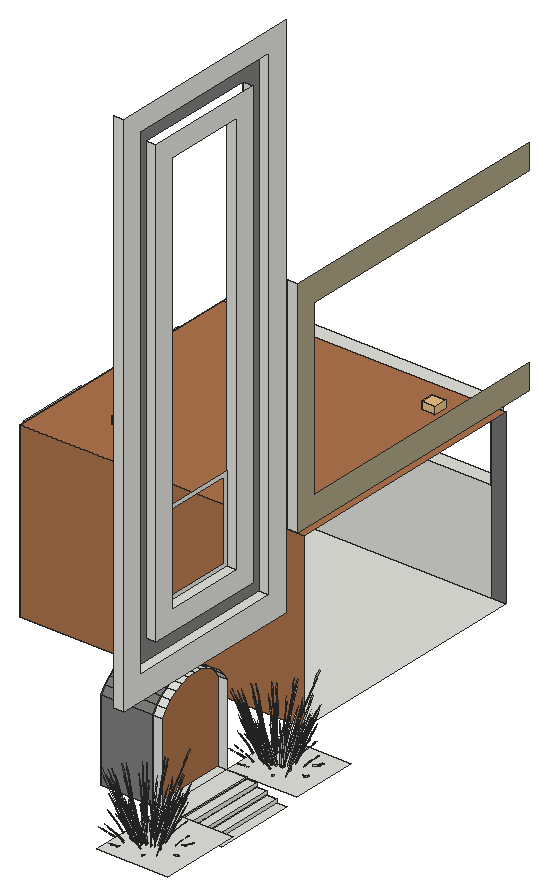
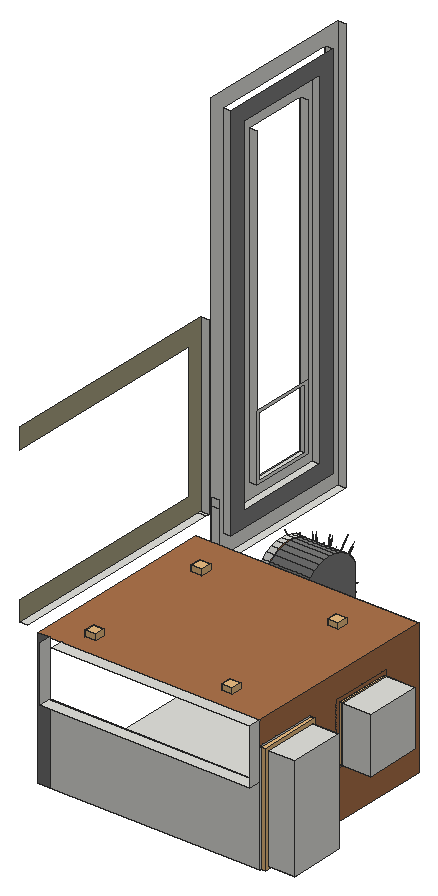
# SketchUp Ruby script. Lengths in inches.
U = 1.inch
M = Sketchup.active_model
def pt(a) = Geom::Point3d.new(a.map { |v| v * U })
def face(e, loops, mat)
  f = e.add_face(loops[0].map { |a| pt(a) })
  loops[1..].each { |l| e.add_face(l.map { |a| pt(a) }).erase! }
  f.material = f.back_material = mat if mat
  f
end
# faces: each face lists its corners as indices into pts; further lists are holes
def faces(e, pts, list, mat = nil) = list.each { |f| face(e, (f[0].is_a?(Array) ? f : [f]).map { |l| l.map { |i| pts[i] } }, mat) }
# xy, xz, yz: faces in a plane at the given z, y or x. An outline is a flat list of corners, or four numbers for a rectangle; further outlines are holes
def ring(l) = l.size == 4 ? [[l[0], l[1]], [l[2], l[1]], [l[2], l[3]], [l[0], l[3]]] : l.each_slice(2).to_a
def flat(e, list, mat, &to3) = list.each { |f| face(e, (f[0].is_a?(Array) ? f : [f]).map { |l| ring(l).map { |u, v| to3.(u, v) } }, mat) }
def xy(e, z, list, mat = nil) = flat(e, list, mat) { |x, y| [x, y, z] }
def xz(e, y, list, mat = nil) = flat(e, list, mat) { |x, z| [x, y, z] }
def yz(e, x, list, mat = nil) = flat(e, list, mat) { |y, z| [x, y, z] }
def lines(e, pts, list) = list.each { |a, b| e.add_line(pt(pts[a]), pt(pts[b])) }
# prism: a flat outline (further loops are holes) pulled along v
def prism(e, loops, v, mat = nil)
  f = face(e, loops, mat); d = Geom::Vector3d.new(v.map { |x| x * U })
  f.pushpull(f.normal.samedirection?(d) ? d.length : -d.length)
end
def box(e, o, s, mat = nil) = prism(e, [[o, [o[0] + s[0], o[1], o[2]], [o[0] + s[0], o[1] + s[1], o[2]], [o[0], o[1] + s[1], o[2]]]], [0, 0, s[2]], mat)
def at(x, y, z, deg = 0) = Geom::Transformation.translation(pt([x, y, z])) * Geom::Transformation.rotation(ORIGIN, Z_AXIS, deg.degrees)
def axes(o, x, y, z) = Geom::Transformation.new([*x, 0, *y, 0, *z, 0, *pt(o).to_a, 1])
def part(name) = M.definitions.add(name)
# library, detail: a bought-in or finely detailed component or shape, given as its bounding box
def library(name, o, s) = part(name).tap { |d| box(d.entities, o, s) }
def detail(e, o, s) = box(e.add_group.entities, o, s)
def put(e, d, t, mat = nil) = e.add_instance(d, t).tap { |i| i.material = mat if mat }
def group(e, t, mat = nil) = e.add_group.tap { |g| g.transformation = t; g.material = mat if mat }.entities
root = M.entities
M.materials.add("LightPink_Translucent").color = [144, 107, 117]
M.materials["LightPink_Translucent"].alpha = 0.75
M.materials.add("M05_Graphite_Haze").color = [114, 114, 114]
M.materials.add("ThomThom - Beard1").color = [170, 163, 131]
M.materials.add("ThomThom - Waistcoat2").color = [127, 127, 126]
M.materials.add("Wood_Veneer_15_1K").color = [173, 116, 75]
c1 = part("blade")
p = [[2.15,0.21,22],[0,0.17,0],[0.09,0.45,0],[2.18,0.31,22],[2.29,0.31,22],[0.38,0.45,0],
  [2.48,0.24,33],[2.49,0.24,33],[2.48,0.22,33]]
faces(c1.entities,p,[[0,1,2,3],[4,5,2,3],[6,3,4,7],[8,0,3,6]])
c2 = part("seeds")
p = [[0.3,-0.1,1.38],[-0.01,-0.03,1.59],[-0.01,-0.03,0.03],[0.14,-0.07,-0.07],[0.29,-0.03,3],[0.15,0.01,3.11]]
faces(c2.entities,p,[[0,1,2,3],[1,0,4,5]],"LightPink_Translucent")
c3 = part("blade with seeds")
put(c3.entities,c1,at(0,0,0))
put(c3.entities,c2,axes([2.4,0.25,30.99],[1.5799,-0.05474,1.17369],[-0.12525,1.92788,0.29478],[-0.07173,-0.02425,1.56792]))
c4 = library("porta+4",[0.2,-5.42,1.33],[46.55,4.72,83.21])
c5 = library("Group\#3",[0,0,0],[2.375,32.33,79.75])
c6 = library("Sphere Light\#7",[-4.125,-4.125,-4.125],[8.25,8.25,8.25])
c7 = library("Sphere Light\#8",[-4,-4,-4],[8,8,8])
c8 = library("Sphere Light\#9",[-4,-4,-4],[8,8,8])
c9 = library("Sphere Light\#10",[-4,-4,-4],[8,8,8])
xy(root,4.51,[[503.8,48,509.78,96],[509.78,48,515.75,96]])
xy(root,6.76,[[497.83,48,503.8,96],[503.8,48,509.78,96]])
xy(root,9,[[312,153,480,303]])
xy(root,9.01,[[491.86,48,497.83,96],[497.83,48,503.8,96]])
xy(root,11.26,[[480,48,491.86,96],[491.86,48,497.83,96]])
xy(root,12,[[480,0,521.72,0,521.72,48,491.86,48,491.86,96,480,96],[474.67,48,480,96],[480,96,521.72,136.05],[288,258,312,300]])
xy(root,12,[[444,48,474.67,96]],"ThomThom - Waistcoat2")
xy(root,48,[[288,186,312,228]])
xy(root,69,[[312,303,471,312]])
xy(root,81.33,[[480,12,486,132]])
xy(root,90,[[288,186,312,228],[288,258,312,300]])
xy(root,96,[[480,24,486,120]])
xy(root,108,[[480,36,486,108]])
xy(root,111,[[312,303,462,312]])
xy(root,111,[[[312,153,480,303],[348.15,280.73,349.1875,280.78,350.18,281.11,351.06,281.68,351.75,282.46,352.23,283.39,352.44,284.41,352.38,285.45,352.06,286.44,351.49,287.32,350.71,288.02,349.78,288.49,348.76,288.7,347.71,288.65,346.72,288.32,345.85,287.75,345.15,286.97,344.68,286.04,344.46,285.02,344.52,283.98,344.85,282.99,345.42,282.11,346.19,281.41,347.125,280.94],[348.15,180.38,349.1875,180.4375,350.18,180.76,351.06,181.33,351.75,182.11,352.23,183.04,352.44,184.06,352.38,185.11,352.06,186.1,351.49,186.97,350.71,187.67,349.78,188.14,348.76,188.36,347.71,188.3,346.72,187.98,345.85,187.41,345.15,186.63,344.68,185.7,344.46,184.68,344.52,183.63,344.85,182.64,345.42,181.77,346.19,181.07,347.125,180.6],[451.37,180.38,452.41,180.4375,453.4,180.76,454.28,181.33,454.97,182.11,455.45,183.04,455.66,184.06,455.61,185.11,455.28,186.1,454.71,186.97,453.93,187.67,453,188.14,451.98,188.36,450.9375,188.3,449.94,187.98,449.07,187.41,448.37,186.63,447.9,185.7,447.69,184.68,447.74,183.63,448.07,182.64,448.64,181.77,449.42,181.07,450.35,180.6],[451.37,280.73,452.41,280.78,453.4,281.11,454.28,281.68,454.97,282.46,455.45,283.39,455.66,284.41,455.61,285.45,455.28,286.44,454.71,287.32,453.93,288.02,453,288.49,451.98,288.7,450.9375,288.65,449.94,288.32,449.07,287.75,448.37,286.97,447.9,286.04,447.69,285.02,447.74,283.98,448.07,282.99,448.64,282.11,449.42,281.41,450.35,280.94]],[348.15,180.38,347.125,180.6,346.19,181.07,345.42,181.77,344.85,182.64,344.52,183.63,344.46,184.68,344.68,185.7,345.15,186.63,345.85,187.41,346.72,187.98,347.71,188.3,348.76,188.36,349.78,188.14,350.71,187.67,351.49,186.97,352.06,186.1,352.38,185.11,352.44,184.06,352.23,183.04,351.75,182.11,351.06,181.33,350.18,180.76,349.1875,180.4375],[451.37,180.38,450.35,180.6,449.42,181.07,448.64,181.77,448.07,182.64,447.74,183.63,447.69,184.68,447.9,185.7,448.37,186.63,449.07,187.41,449.94,187.98,450.9375,188.3,451.98,188.36,453,188.14,453.93,187.67,454.71,186.97,455.28,186.1,455.61,185.11,455.66,184.06,455.45,183.04,454.97,182.11,454.28,181.33,453.4,180.76,452.41,180.4375],[348.15,280.73,347.125,280.94,346.19,281.41,345.42,282.11,344.85,282.99,344.52,283.98,344.46,285.02,344.68,286.04,345.15,286.97,345.85,287.75,346.72,288.32,347.71,288.65,348.76,288.7,349.78,288.49,350.71,288.02,351.49,287.32,352.06,286.44,352.38,285.45,352.44,284.41,352.23,283.39,351.75,282.46,351.06,281.68,350.18,281.11,349.1875,280.78],[451.37,280.73,450.35,280.94,449.42,281.41,448.64,282.11,448.07,282.99,447.74,283.98,447.69,285.02,447.9,286.04,448.37,286.97,449.07,287.75,449.94,288.32,450.9375,288.65,451.98,288.7,453,288.49,453.93,288.02,454.71,287.32,455.28,286.44,455.61,285.45,455.66,284.41,455.45,283.39,454.97,282.46,454.28,281.68,453.4,281.11,452.41,280.78]],"Wood_Veneer_15_1K")
xy(root,120,[[480,48,486,96],[480,141,486,144],[480,144,486,312]])
xz(root,12,[[480,81.33,486,396]])
xz(root,24,[[480,96,486,384]])
xz(root,36,[[480,108,486,372]])
xz(root,48,[[474.67,12,480,60],[480,120,486,360]])
xz(root,48,[[444,12,474.67,60]],"ThomThom - Waistcoat2")
xz(root,96,[[503.8,4.51,509.78,6.76],[497.83,6.76,503.8,9.01],[491.86,9.01,497.83,11.26],[480,11.26,491.86,12],[474.67,12,480,60],
  [480,120,486,360]])
xz(root,96,[[444,12,474.67,60]],"ThomThom - Waistcoat2")
xz(root,108,[[480,108,486,372]])
xz(root,120,[[480,96,486,384]])
xz(root,132,[[480,81.33,486,120],[480,120,486,126]])
xz(root,141,[[480,120,486,252]])
xz(root,153,[[312,9,480,111]],"Wood_Veneer_15_1K")
xz(root,186,[[288,48,312,90]])
xz(root,228,[[288,48,312,90]])
xz(root,258,[[288,12,312,90]])
xz(root,300,[[288,12,312,90]])
xz(root,303,[[312,9,471,69]])
xz(root,303,[[471,9,480,111]],"M05_Graphite_Haze")
yz(root,288,[[258,12,300,90],[186,48,228,90]])
yz(root,312,[[[255,9,303,93],[258,12,300,90]],[303,69,312,111]])
yz(root,312,[[[153,9,255,9,255,93,303,93,303,111,153,111],[183,45,231,93]],[[183,45,231,93],[186,48,228,90]]],"Wood_Veneer_15_1K")
yz(root,444,[[48,12,96,12,96,60,93.26,64,89.86,67.47,85.9,70.28,81.52,72.35,76.83,73.62,72,74.05,67.17,73.62,62.48,72.35,58.1,70.28,54.14,67.47,50.74,64,48,60]],"ThomThom - Waistcoat2")
yz(root,471,[[303,69,312,111]])
yz(root,474.67,[[48,12,96,12,96,60,93.26,64,89.86,67.47,85.9,70.28,81.52,72.35,76.83,73.62,72,74.05,67.17,73.62,62.48,72.35,58.1,70.28,54.14,67.47,50.74,64,48,60]],"Wood_Veneer_15_1K")
yz(root,480,[[[48,120,96,170.38],[50,122,94,168.38]]])
yz(root,480,[[[24,96,120,384],[36,108,108,372]]],"ThomThom - Waistcoat2")
yz(root,486,[[[12,81.33,132,396],[24,96,120,384]],[[36,108,108,372],[48,120,96,360]]])
yz(root,486,[[141,120,312,120,312,135,153,135,153,237,312,237,312,252,141,252]],"ThomThom - Beard1")
yz(root,491.86,[[48,9.01,96,11.26],[48,11.26,96,11.38],[48,11.38,96,12]])
yz(root,497.83,[[48,6.76,96,9.01],[48,9.01,96,11.26]])
yz(root,503.8,[[48,4.51,96,6.76],[48,6.76,96,9.01]])
yz(root,509.78,[[48,4.51,96,6.76]])
p = [[444,50.74,64],[474.67,50.74,64],[474.67,48,60],[444,48,60],[480,50.74,64],[480,48,60],
  [444,96,60],[474.67,96,60],[474.67,93.26,64],[444,93.26,64],[480,96,60],[480,93.26,64],
  [444,54.14,67.47],[474.67,54.14,67.47],[480,54.14,67.47],[474.67,89.86,67.47],[444,89.86,67.47],[480,89.86,67.47],
  [444,58.1,70.28],[474.67,58.1,70.28],[480,58.1,70.28],[474.67,85.9,70.28],[444,85.9,70.28],[480,85.9,70.28],
  [444,62.48,72.35],[474.67,62.48,72.35],[480,62.48,72.35],[474.67,81.52,72.35],[444,81.52,72.35],[480,81.52,72.35],
  [444,67.17,73.62],[474.67,67.17,73.62],[480,67.17,73.62],[474.67,76.83,73.62],[444,76.83,73.62],[480,76.83,73.62],
  [444,72,74.05],[474.67,72,74.05],[480,72,74.05],[312,303,105],[312,303,9],[312,255,9]]
faces(root,p,[[0,1,2,3],[6,7,8,9],[12,13,1,0],[9,8,15,16],[18,19,13,12],[16,15,21,22],[24,25,19,18],[22,21,27,28],
  [30,31,25,24],[28,27,33,34],[36,37,31,30],[34,33,37,36]],"ThomThom - Waistcoat2")
faces(root,p,[[4,5,2,1],[10,11,8,7],[14,4,1,13],[11,17,15,8],[20,14,13,19],[17,23,21,15],[26,20,19,25],[23,29,27,21],
  [32,26,25,31],[29,35,33,27],[38,32,31,37],[35,38,37,33]])
lines(root,p,[[39,40],[40,41]])
put(root,c3,axes([496.09,122.125,5.03],[0.06562,-1.05324,-0.1216],[1.2424,0.02879,-0.67495],[0.4785,0.07316,1.02557]))
put(root,c3,axes([486.79,118.08,5.03],[0.6166,0.93779,-0.1216],[-1.09436,0.46085,-0.67495],[-0.46117,0.12373,1.02557]))
put(root,c3,axes([495.96,116.03,5.03],[-1.34686,-0.05131,-0.1216],[0.03681,-0.97156,-0.67495],[0.09356,-0.37418,1.02557]))
put(root,c3,axes([497.47,120.18,5.03],[-0.6166,-0.93779,-0.1216],[1.09436,-0.46085,-0.67495],[0.46117,-0.12373,1.02557]))
put(root,c3,axes([490.79,123.31,5.03],[1.19922,-0.48218,-0.1216],[0.58932,0.85579,-0.67495],[0.15822,0.36063,1.02557]))
put(root,c3,axes([488.17,116.13,5.03],[-0.06562,1.05324,-0.1216],[-1.2424,-0.02879,-0.67495],[-0.4785,-0.07316,1.02557]))
put(root,c3,axes([493.64,123.27,5.03],[0.73026,-0.88648,-0.1216],[1.05755,0.51071,-0.67495],[0.36761,0.25045,1.02557]))
put(root,c3,axes([486.83,120.31,5.03],[1.1336,0.57106,-0.1216],[-0.65308,0.827,-0.67495],[-0.32027,0.28747,1.02557]))
put(root,c3,axes([493.47,114.95,5.03],[-1.19922,0.48218,-0.1216],[-0.58932,-0.85579,-0.67495],[-0.15822,-0.36063,1.02557]))
put(root,c3,axes([497.42,117.95,5.03],[-1.1336,-0.57106,-0.1216],[0.65308,-0.827,-0.67495],[0.32027,-0.28747,1.02557]))
put(root,c3,axes([496.09,26.125,5.03],[0.06562,-1.05324,-0.1216],[1.2424,0.02879,-0.67495],[0.4785,0.07316,1.02557]))
put(root,c3,axes([486.79,22.08,5.03],[0.6166,0.93779,-0.1216],[-1.09436,0.46085,-0.67495],[-0.46117,0.12373,1.02557]))
put(root,c3,axes([495.96,20.03,5.03],[-1.34686,-0.05131,-0.1216],[0.03681,-0.97156,-0.67495],[0.09356,-0.37418,1.02557]))
put(root,c3,axes([497.47,24.18,5.03],[-0.6166,-0.93779,-0.1216],[1.09436,-0.46085,-0.67495],[0.46117,-0.12373,1.02557]))
put(root,c3,axes([490.79,27.31,5.03],[1.19922,-0.48218,-0.1216],[0.58932,0.85579,-0.67495],[0.15822,0.36063,1.02557]))
put(root,c3,axes([488.17,20.13,5.03],[-0.06562,1.05324,-0.1216],[-1.2424,-0.02879,-0.67495],[-0.4785,-0.07316,1.02557]))
put(root,c3,axes([493.64,27.27,5.03],[0.73026,-0.88648,-0.1216],[1.05755,0.51071,-0.67495],[0.36761,0.25045,1.02557]))
put(root,c3,axes([486.83,24.31,5.03],[1.1336,0.57106,-0.1216],[-0.65308,0.827,-0.67495],[-0.32027,0.28747,1.02557]))
put(root,c3,axes([493.47,18.95,5.03],[-1.19922,0.48218,-0.1216],[-0.58932,-0.85579,-0.67495],[-0.15822,-0.36063,1.02557]))
put(root,c3,axes([497.42,21.95,5.03],[-1.1336,-0.57106,-0.1216],[0.65308,-0.827,-0.67495],[0.32027,-0.28747,1.02557]))
put(root,c3,axes([494.47,118.04,4.47],[-1.05895,-0.53811,1.38283],[1.11816,-0.83781,0.59665],[0.34166,0.5049,1.33663]))
put(root,c3,axes([494.47,22.04,4.47],[-1.05895,-0.53811,1.38283],[1.11816,-0.83781,0.59665],[0.34166,0.5049,1.33663]))
put(root,c3,axes([485.5,23.02,4.72],[-0.20012,0.13446,1.74944],[0.01702,0.98243,-0.27667],[-0.45871,0.12776,0.14031]))
put(root,c3,axes([500.82,22.71,4.72],[0.17006,-0.15775,1.74944],[-0.21766,-0.96766,-0.27667],[0.42669,-0.18347,0.14031]))
put(root,c3,axes([497.17,25.49,4.72],[0.26289,-0.01751,1.74944],[0.72108,-0.8046,-0.27667],[0.46761,0.10621,0.14031]))
put(root,c3,axes([497.18,18.49,4.72],[-0.01183,-0.20612,1.74944],[-0.99913,-0.59572,-0.27667],[0.15447,-0.36112,0.14031]))
put(root,c3,axes([485.53,26.69,4.72],[-0.03046,0.20495,1.74944],[0.86449,0.71297,-0.27667],[-0.22632,0.33716,0.14031]))
put(root,c3,axes([490.51,29.22,4.72],[0.15534,0.16677,1.74944],[1.25362,0.06552,-0.27667],[0.12606,0.3678,0.14031]))
put(root,c3,axes([491.5625,16.71,4.72],[-0.18744,-0.14521,1.74944],[-1.25089,0.09206,-0.27667],[-0.19964,-0.34731,0.14031]))
put(root,c3,axes([487.46,18.31,4.72],[-0.26368,-0.00731,1.74944],[-0.83946,0.73103,-0.27667],[-0.44791,-0.14937,0.14031]))
put(root,c3,axes([485.5,119.02,4.72],[-0.20012,0.13446,1.74944],[0.01702,0.98243,-0.27667],[-0.45871,0.12776,0.14031]))
put(root,c3,axes([500.82,118.71,4.72],[0.17006,-0.15775,1.74944],[-0.21766,-0.96766,-0.27667],[0.42669,-0.18347,0.14031]))
put(root,c3,axes([497.17,121.49,4.72],[0.26289,-0.01751,1.74944],[0.72108,-0.8046,-0.27667],[0.46761,0.10621,0.14031]))
put(root,c3,axes([497.18,114.49,4.72],[-0.01183,-0.20612,1.74944],[-0.99913,-0.59572,-0.27667],[0.15447,-0.36112,0.14031]))
put(root,c3,axes([485.53,122.69,4.72],[-0.03046,0.20495,1.74944],[0.86449,0.71297,-0.27667],[-0.22632,0.33716,0.14031]))
put(root,c3,axes([490.51,125.22,4.72],[0.15534,0.16677,1.74944],[1.25362,0.06552,-0.27667],[0.12606,0.3678,0.14031]))
put(root,c3,axes([491.5625,112.71,4.72],[-0.18744,-0.14521,1.74944],[-1.25089,0.09206,-0.27667],[-0.19964,-0.34731,0.14031]))
put(root,c3,axes([487.46,114.31,4.72],[-0.26368,-0.00731,1.74944],[-0.83946,0.73103,-0.27667],[-0.44791,-0.14937,0.14031]))
put(root,c3,axes([486.45,18.93,4.71],[0.09085,0.10335,1.77383],[-0.43798,0.92907,-0.16761],[-0.44357,0.00672,0.31391]))
put(root,c3,axes([490.28,16.23,4.71],[-0.02286,0.12414,1.77383],[-1.12758,0.45052,-0.16761],[-0.33182,-0.23029,0.31391]))
put(root,c3,axes([492.68,28.01,4.71],[0.00363,-0.12539,1.77383],[1.0502,-0.55319,-0.16761],[0.36479,0.19745,0.31391]))
put(root,c3,axes([483.28,24.01,4.71],[0.1564,0.02778,1.77383],[0.48382,0.91506,-0.16761],[-0.32016,0.24017,0.31391]))
put(root,c3,axes([500.22,21.7,4.71],[-0.16006,-0.00787,1.77383],[-0.66468,-0.8428,-0.16761],[0.26693,-0.27711,0.31391]))
put(root,c3,axes([499.92,26.96,4.71],[-0.11081,-0.09067,1.77383],[0.2424,-0.97188,-0.16761],[0.43649,-0.06209,0.31391]))
put(root,c3,axes([485.4375,28.79,4.71],[0.13903,-0.06253,1.77383],[1.14912,0.41591,-0.16761],[-0.027,0.34629,0.31391]))
put(root,c3,axes([496.92,17.75,4.71],[-0.12446,0.07911,1.77383],[-1.21937,-0.26689,-0.16761],[-0.04414,-0.34521,0.31391]))
put(root,c3,axes([486.45,114.93,4.71],[0.09085,0.10335,1.77383],[-0.43798,0.92907,-0.16761],[-0.44357,0.00672,0.31391]))
put(root,c3,axes([490.28,112.23,4.71],[-0.02286,0.12414,1.77383],[-1.12758,0.45052,-0.16761],[-0.33182,-0.23029,0.31391]))
put(root,c3,axes([492.68,124.01,4.71],[0.00363,-0.12539,1.77383],[1.0502,-0.55319,-0.16761],[0.36479,0.19745,0.31391]))
put(root,c3,axes([483.28,120.01,4.71],[0.1564,0.02778,1.77383],[0.48382,0.91506,-0.16761],[-0.32016,0.24017,0.31391]))
put(root,c3,axes([500.22,117.7,4.71],[-0.16006,-0.00787,1.77383],[-0.66468,-0.8428,-0.16761],[0.26693,-0.27711,0.31391]))
put(root,c3,axes([499.92,122.96,4.71],[-0.11081,-0.09067,1.77383],[0.2424,-0.97188,-0.16761],[0.43649,-0.06209,0.31391]))
put(root,c3,axes([485.4375,124.79,4.71],[0.13903,-0.06253,1.77383],[1.14912,0.41591,-0.16761],[-0.027,0.34629,0.31391]))
put(root,c3,axes([496.92,113.75,4.71],[-0.12446,0.07911,1.77383],[-1.21937,-0.26689,-0.16761],[-0.04414,-0.34521,0.31391]))
put(root,c3,axes([488.3,122.22,5.4],[1.34686,0.05131,-0.13498],[-0.03681,0.97156,-0.74919],[-0.09356,0.37418,1.13838]))
put(root,c3,axes([488.3,26.22,5.4],[1.34686,0.05131,-0.13498],[-0.03681,0.97156,-0.74919],[-0.09356,0.37418,1.13838]))
put(root,c3,axes([490.6,18.59,5.43],[-0.81789,0.99285,-0.13619],[-1.18445,-0.572,-0.75594],[-0.41173,-0.28051,1.14864]))
put(root,c3,axes([490.6,114.59,5.43],[-0.81789,0.99285,-0.13619],[-1.18445,-0.572,-0.75594],[-0.41173,-0.28051,1.14864]))
put(root,c3,axes([490.35,114.66,4.73],[0.55698,-0.6579,0.0643],[0.79316,0.38303,0.50621],[-0.25643,-0.21093,0.77189]))
put(root,c3,axes([490.82,123.69,4.73],[-0.90301,0.35198,0.0643],[-0.44199,-0.64184,0.50621],[0.08721,0.28293,0.77189]))
put(root,c3,axes([497.84,117.74,4.73],[0.8413,0.43556,0.0643],[-0.48981,0.62025,0.50621],[0.26973,-0.20053,0.77189]))
put(root,c3,axes([497.96,120.15,4.73],[0.4501,0.70615,0.0643],[-0.82077,0.34564,0.50621],[0.36181,-0.0682,0.77189]))
put(root,c3,axes([487.73,115.96,4.73],[0.06171,-0.78753,0.0643],[0.9318,0.02159,0.50621],[-0.35694,-0.08241,0.77189]))
put(root,c3,axes([496.18,115.69,4.73],[1.00708,0.04826,0.0643],[-0.02761,0.72867,0.50621],[0.10538,-0.27912,0.77189]))
put(root,c3,axes([496.53,122.3,4.73],[-0.06171,0.78753,0.0643],[-0.9318,-0.02159,0.50621],[0.35694,0.08241,0.77189]))
put(root,c3,axes([486.42,120.52,4.73],[-0.8413,-0.43556,0.0643],[0.48981,-0.62025,0.50621],[-0.26973,0.20053,0.77189]))
put(root,c3,axes([493.44,114.57,4.73],[0.90301,-0.35198,0.0643],[0.44199,0.64184,0.50621],[-0.08721,-0.28293,0.77189]))
put(root,c3,axes([486.29,118.1,4.73],[-0.4501,-0.70615,0.0643],[0.82077,-0.34564,0.50621],[-0.36181,0.0682,0.77189]))
put(root,c3,axes([493.91,123.59,4.73],[-0.55698,0.6579,0.0643],[-0.79316,-0.38303,0.50621],[0.25643,0.21093,0.77189]))
put(root,c3,axes([488.07,122.57,4.73],[-1.00708,-0.04826,0.0643],[0.02761,-0.72867,0.50621],[-0.10538,0.27912,0.77189]))
put(root,c3,axes([490.35,18.66,4.73],[0.55698,-0.6579,0.0643],[0.79316,0.38303,0.50621],[-0.25643,-0.21093,0.77189]))
put(root,c3,axes([490.82,27.69,4.73],[-0.90301,0.35198,0.0643],[-0.44199,-0.64184,0.50621],[0.08721,0.28293,0.77189]))
put(root,c3,axes([497.84,21.74,4.73],[0.8413,0.43556,0.0643],[-0.48981,0.62025,0.50621],[0.26973,-0.20053,0.77189]))
put(root,c3,axes([497.96,24.15,4.73],[0.4501,0.70615,0.0643],[-0.82077,0.34564,0.50621],[0.36181,-0.0682,0.77189]))
put(root,c3,axes([487.73,19.96,4.73],[0.06171,-0.78753,0.0643],[0.9318,0.02159,0.50621],[-0.35694,-0.08241,0.77189]))
put(root,c3,axes([496.18,19.69,4.73],[1.00708,0.04826,0.0643],[-0.02761,0.72867,0.50621],[0.10538,-0.27912,0.77189]))
put(root,c3,axes([496.53,26.3,4.73],[-0.06171,0.78753,0.0643],[-0.9318,-0.02159,0.50621],[0.35694,0.08241,0.77189]))
put(root,c3,axes([486.42,24.52,4.73],[-0.8413,-0.43556,0.0643],[0.48981,-0.62025,0.50621],[-0.26973,0.20053,0.77189]))
put(root,c3,axes([493.44,18.57,4.73],[0.90301,-0.35198,0.0643],[0.44199,0.64184,0.50621],[-0.08721,-0.28293,0.77189]))
put(root,c3,axes([486.29,22.1,4.73],[-0.4501,-0.70615,0.0643],[0.82077,-0.34564,0.50621],[-0.36181,0.0682,0.77189]))
put(root,c3,axes([493.91,27.59,4.73],[-0.55698,0.6579,0.0643],[-0.79316,-0.38303,0.50621],[0.25643,0.21093,0.77189]))
put(root,c3,axes([488.07,26.57,4.73],[-1.00708,-0.04826,0.0643],[0.02761,-0.72867,0.50621],[-0.10538,0.27912,0.77189]))
put(root,c3,axes([493.12,114.63,4.73],[1.20755,0.27075,0.48003],[-0.41292,0.89013,0.3958],[-0.07257,-0.35005,0.9933]))
put(root,c3,axes([496.61,122.05,4.73],[-0.90362,0.68241,0.48003],[-0.77932,-0.72471,0.3958],[0.42395,0.12588,0.9933]))
put(root,c3,axes([497.88,119.9,4.73],[-0.34623,0.9443,0.48003],[-1.13828,-0.3229,0.3958],[0.44763,-0.05675,0.9933]))
put(root,c3,axes([486.65,120.7,4.73],[-0.30393,-0.95317,0.48003],[1.19224,-0.16542,0.3958],[-0.35138,0.22417,0.9933]))
put(root,c3,axes([488.4,122.63,4.73],[-0.87265,-0.70663,0.48003],[0.92674,-0.60943,0.3958],[-0.16097,0.33153,0.9933]))
put(root,c3,axes([495.86,115.625,4.73],[0.87265,0.70663,0.48003],[-0.92674,0.60943,0.3958],[0.16097,-0.33153,0.9933]))
put(root,c3,axes([486.38,118.35,4.73],[0.34623,-0.9443,0.48003],[1.13828,0.3229,0.3958],[-0.44763,0.05675,0.9933]))
put(root,c3,axes([497.6,117.55,4.73],[0.30393,0.95317,0.48003],[-1.19224,0.16542,0.3958],[0.35138,-0.22417,0.9933]))
put(root,c3,axes([494.14,123.41,4.73],[-1.21888,0.23767,0.48003],[-0.21154,-0.93233,0.3958],[0.28666,0.27478,0.9933]))
put(root,c3,axes([493.12,18.63,4.73],[1.20755,0.27075,0.48003],[-0.41292,0.89013,0.3958],[-0.07257,-0.35005,0.9933]))
put(root,c3,axes([496.61,26.05,4.73],[-0.90362,0.68241,0.48003],[-0.77932,-0.72471,0.3958],[0.42395,0.12588,0.9933]))
put(root,c3,axes([497.88,23.9,4.73],[-0.34623,0.9443,0.48003],[-1.13828,-0.3229,0.3958],[0.44763,-0.05675,0.9933]))
put(root,c3,axes([486.65,24.7,4.73],[-0.30393,-0.95317,0.48003],[1.19224,-0.16542,0.3958],[-0.35138,0.22417,0.9933]))
put(root,c3,axes([488.4,26.63,4.73],[-0.87265,-0.70663,0.48003],[0.92674,-0.60943,0.3958],[-0.16097,0.33153,0.9933]))
put(root,c3,axes([495.86,19.625,4.73],[0.87265,0.70663,0.48003],[-0.92674,0.60943,0.3958],[0.16097,-0.33153,0.9933]))
put(root,c3,axes([486.38,22.35,4.73],[0.34623,-0.9443,0.48003],[1.13828,0.3229,0.3958],[-0.44763,0.05675,0.9933]))
put(root,c3,axes([497.6,21.55,4.73],[0.30393,0.95317,0.48003],[-1.19224,0.16542,0.3958],[0.35138,-0.22417,0.9933]))
put(root,c3,axes([494.14,27.41,4.73],[-1.21888,0.23767,0.48003],[-0.21154,-0.93233,0.3958],[0.28666,0.27478,0.9933]))
put(root,c3,axes([491.15,122.97,5.05],[0.36946,-0.79643,0.35414],[1.07787,0.23229,-0.4572],[0.09883,0.32066,0.87481]))
put(root,c3,axes([493.11,115.29,5.05],[-0.36946,0.79643,0.35414],[-1.07787,-0.23229,-0.4572],[-0.09883,-0.32066,0.87481]))
put(root,c3,axes([495.89,121.71,5.05],[-0.69728,-0.64842,0.35414],[0.79619,-0.61382,-0.4572],[0.40453,0.09339,0.87481]))
put(root,c3,axes([497.04,119.89,5.05],[-1.01846,-0.28891,0.35414],[0.29705,-0.84289,-0.4572],[0.41005,-0.07729,0.87481]))
put(root,c3,axes([488.36,116.55,5.05],[0.69728,0.64842,0.35414],[-0.79619,0.61382,-0.4572],[-0.40453,-0.09339,0.87481]))
put(root,c3,axes([488.83,122.07,5.05],[0.82919,-0.54528,0.35414],[0.78493,0.62262,-0.4572],[-0.11943,0.31634,0.87481]))
put(root,c3,axes([487.39,120.39,5.05],[1.06674,-0.14801,0.35414],[0.28168,0.84611,-0.4572],[-0.30569,0.22726,0.87481]))
put(root,c3,axes([493.74,122.84,5.05],[-0.18927,-0.83419,0.35414],[1.08199,-0.22027,-0.4572],[0.29062,0.23905,0.87481]))
put(root,c3,axes([496.87,117.87,5.05],[-1.06674,0.14801,0.35414],[-0.28168,-0.84611,-0.4572],[0.30569,-0.22726,0.87481]))
put(root,c3,axes([487.22,118.36,5.05],[1.01846,0.28891,0.35414],[-0.29705,0.84289,-0.4572],[-0.41005,0.07729,0.87481]))
put(root,c3,axes([495.43,116.18,5.05],[-0.82919,0.54528,0.35414],[-0.78493,-0.62262,-0.4572],[0.11943,-0.31634,0.87481]))
put(root,c3,axes([490.52,115.42,5.05],[0.18927,0.83419,0.35414],[-1.08199,0.22027,-0.4572],[-0.29062,-0.23905,0.87481]))
put(root,c3,axes([491.15,26.97,5.05],[0.36946,-0.79643,0.35414],[1.07787,0.23229,-0.4572],[0.09883,0.32066,0.87481]))
put(root,c3,axes([493.11,19.29,5.05],[-0.36946,0.79643,0.35414],[-1.07787,-0.23229,-0.4572],[-0.09883,-0.32066,0.87481]))
put(root,c3,axes([495.89,25.71,5.05],[-0.69728,-0.64842,0.35414],[0.79619,-0.61382,-0.4572],[0.40453,0.09339,0.87481]))
put(root,c3,axes([497.04,23.89,5.05],[-1.01846,-0.28891,0.35414],[0.29705,-0.84289,-0.4572],[0.41005,-0.07729,0.87481]))
put(root,c3,axes([488.36,20.55,5.05],[0.69728,0.64842,0.35414],[-0.79619,0.61382,-0.4572],[-0.40453,-0.09339,0.87481]))
put(root,c3,axes([488.83,26.07,5.05],[0.82919,-0.54528,0.35414],[0.78493,0.62262,-0.4572],[-0.11943,0.31634,0.87481]))
put(root,c3,axes([487.39,24.39,5.05],[1.06674,-0.14801,0.35414],[0.28168,0.84611,-0.4572],[-0.30569,0.22726,0.87481]))
put(root,c3,axes([493.74,26.84,5.05],[-0.18927,-0.83419,0.35414],[1.08199,-0.22027,-0.4572],[0.29062,0.23905,0.87481]))
put(root,c3,axes([496.87,21.87,5.05],[-1.06674,0.14801,0.35414],[-0.28168,-0.84611,-0.4572],[0.30569,-0.22726,0.87481]))
put(root,c3,axes([487.22,22.36,5.05],[1.01846,0.28891,0.35414],[-0.29705,0.84289,-0.4572],[-0.41005,0.07729,0.87481]))
put(root,c3,axes([495.43,20.18,5.05],[-0.82919,0.54528,0.35414],[-0.78493,-0.62262,-0.4572],[0.11943,-0.31634,0.87481]))
put(root,c3,axes([490.52,19.42,5.05],[0.18927,0.83419,0.35414],[-1.08199,0.22027,-0.4572],[-0.29062,-0.23905,0.87481]))
put(root,c3,axes([491.14,123.625,5.0625],[-1.20755,-0.27075,0.53283],[0.41292,-0.89013,0.43934],[0.07257,0.35005,1.10256]))
put(root,c3,axes([491.14,27.625,5.0625],[-1.20755,-0.27075,0.53283],[0.41292,-0.89013,0.43934],[0.07257,0.35005,1.10256]))
put(root,c3,axes([487.27,115.96,5.09],[1.01205,-0.7643,0.53763],[0.87284,0.81167,0.4433],[-0.47482,-0.14098,1.11249]))
put(root,c3,axes([490.03,114.4375,5.09],[1.36515,-0.26619,0.53763],[0.23692,1.04421,0.4433],[-0.32106,-0.30775,1.11249]))
put(root,c3,axes([487.27,19.96,5.09],[1.01205,-0.7643,0.53763],[0.87284,0.81167,0.4433],[-0.47482,-0.14098,1.11249]))
put(root,c3,axes([490.03,18.4375,5.09],[1.36515,-0.26619,0.53763],[0.23692,1.04421,0.4433],[-0.32106,-0.30775,1.11249]))
put(root,c3,axes([492.6,125.8125,5.65],[0.84686,-0.59414,-0.06488],[0.77596,0.65071,-0.29416],[0.05463,0.18438,0.97024]))
put(root,c3,axes([484.96,122.79,5.65],[1.08141,0.27645,-0.06488],[-0.33265,0.85086,-0.29416],[-0.17688,0.12919,0.97024]))
put(root,c3,axes([492.6,29.8125,5.65],[0.84686,-0.59414,-0.06488],[0.77596,0.65071,-0.29416],[0.05463,0.18438,0.97024]))
put(root,c3,axes([484.96,26.79,5.65],[1.08141,0.27645,-0.06488],[-0.33265,0.85086,-0.29416],[-0.17688,0.12919,0.97024]))
put(root,c4,at(307.72,254.8,7.66,90))
put(root,c5,axes([312.17,228,48],[-0.92105,0,0],[0,-1.29897,0],[0,0,0.52665]))
put(root,c6,at(451.62,184.21,111))
put(root,c7,at(451.67,284.71,111))
put(root,c8,at(348.45,284.71,111))
put(root,c9,at(348.45,184.37,111))
